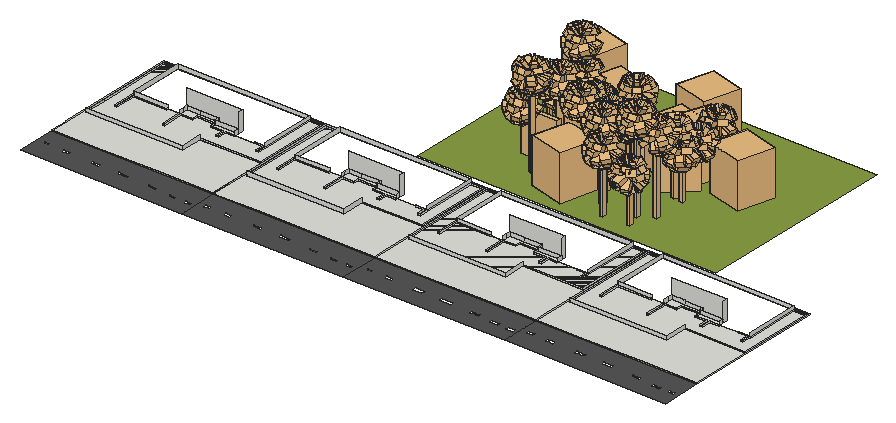
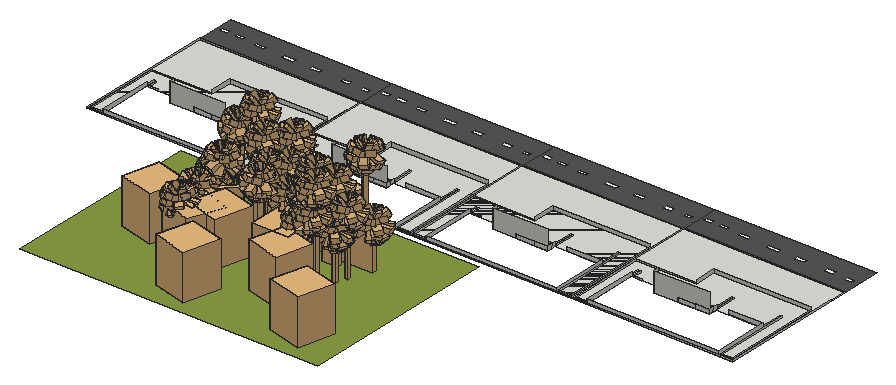
# SketchUp Ruby script. Lengths in inches.
U = 1.inch
M = Sketchup.active_model
def pt(a) = Geom::Point3d.new(a.map { |v| v * U })
def face(e, loops, mat)
  f = e.add_face(loops[0].map { |a| pt(a) })
  loops[1..].each { |l| e.add_face(l.map { |a| pt(a) }).erase! }
  f.material = f.back_material = mat if mat
  f
end
# faces: each face lists its corners as indices into pts; further lists are holes
def faces(e, pts, list, mat = nil) = list.each { |f| face(e, (f[0].is_a?(Array) ? f : [f]).map { |l| l.map { |i| pts[i] } }, mat) }
# xy, xz, yz: faces in a plane at the given z, y or x. An outline is a flat list of corners, or four numbers for a rectangle; further outlines are holes
def ring(l) = l.size == 4 ? [[l[0], l[1]], [l[2], l[1]], [l[2], l[3]], [l[0], l[3]]] : l.each_slice(2).to_a
def flat(e, list, mat, &to3) = list.each { |f| face(e, (f[0].is_a?(Array) ? f : [f]).map { |l| ring(l).map { |u, v| to3.(u, v) } }, mat) }
def xy(e, z, list, mat = nil) = flat(e, list, mat) { |x, y| [x, y, z] }
def xz(e, y, list, mat = nil) = flat(e, list, mat) { |x, z| [x, y, z] }
def yz(e, x, list, mat = nil) = flat(e, list, mat) { |y, z| [x, y, z] }
def lines(e, pts, list) = list.each { |a, b| e.add_line(pt(pts[a]), pt(pts[b])) }
# prism: a flat outline (further loops are holes) pulled along v
def prism(e, loops, v, mat = nil)
  f = face(e, loops, mat); d = Geom::Vector3d.new(v.map { |x| x * U })
  f.pushpull(f.normal.samedirection?(d) ? d.length : -d.length)
end
def box(e, o, s, mat = nil) = prism(e, [[o, [o[0] + s[0], o[1], o[2]], [o[0] + s[0], o[1] + s[1], o[2]], [o[0], o[1] + s[1], o[2]]]], [0, 0, s[2]], mat)
def at(x, y, z, deg = 0) = Geom::Transformation.translation(pt([x, y, z])) * Geom::Transformation.rotation(ORIGIN, Z_AXIS, deg.degrees)
def axes(o, x, y, z) = Geom::Transformation.new([*x, 0, *y, 0, *z, 0, *pt(o).to_a, 1])
def part(name) = M.definitions.add(name)
# library, detail: a bought-in or finely detailed component or shape, given as its bounding box
def library(name, o, s) = part(name).tap { |d| box(d.entities, o, s) }
def detail(e, o, s) = box(e.add_group.entities, o, s)
def put(e, d, t, mat = nil) = e.add_instance(d, t).tap { |i| i.material = mat if mat }
def group(e, t, mat = nil) = e.add_group.tap { |g| g.transformation = t; g.material = mat if mat }.entities
root = M.entities
M.materials.add("COCOLUMBER1").color = [119, 109, 95]
M.materials.add("Color_000").color = [255, 255, 255]
M.materials.add("[0133_Gray]").color = [86, 86, 86]
M.materials.add("[Grass Light Green]").color = [138, 158, 69]
M.materials.add("[Stone_Flagstone_Ashlar]").color = [175, 116, 102]
M.materials.add("[Tile Grey]").color = [168, 168, 168]
c1 = part("Untitled (5)")
xy(c1.entities,0,[[222.04,66.5,231.29,100.5],[222.61,182.28,236.36,226.53],[225.28,357.51,237.28,411.51],[226.57,518.17,239.57,583.92],[233.64,703.93,242.14,755.18],
  [240.05,835.03,248.8,880.53],[239.71,931.55,251.46,972.3]],"Color_000")
xy(c1.entities,0,[[[158.81,26.5625,306.06,993.3125],[226.57,518.17,239.57,583.92],[225.28,357.51,237.28,411.51],[222.61,182.28,236.36,226.53],[239.71,931.55,251.46,972.3],[233.64,703.93,242.14,755.18],[240.05,835.03,248.8,880.53],[222.04,66.5,231.29,100.5]]],"[0133_Gray]")
c2 = library("Palm frond \#1",[-21.27,-0.38,-4.44],[74.64,151.68,26.05])
c3 = part("Palm frond cluster")
put(c3.entities,c2,axes([98.98,59.12,-6.6],[-0.57786,0.81614,0],[-0.81614,-0.57786,0],[0,0,1.8876]))
put(c3.entities,c2,axes([105.83,88.13,9.87],[-0.67944,-0.73373,0],[0.7249,-0.67126,-0.15471],[0.21427,-0.19842,1.86487]))
put(c3.entities,c2,axes([73.46,76.73,-6.83],[1,0,0],[0,0.99443,-0.10543],[0,0.19901,1.87708]))
c4 = part("Palm crown")
put(c4.entities,c2,axes([108.09,116.23,112.23],[0.60444,0.79634,0.02211],[-0.38669,0.31755,-0.86581],[-0.57427,0.42444,0.41215]))
put(c4.entities,c2,axes([136.99,132.05,110.62],[-0.9152,-0.38852,0.10706],[0.08408,-0.44389,-0.89213],[0.32496,-0.66577,0.36188]))
put(c4.entities,c2,axes([122.18,113.8,111.54],[0.08804,0.99481,0.05098],[-0.50379,0.08862,-0.85927],[-0.70852,0.0412,0.41966]))
put(c4.entities,c2,axes([127.99,125.91,114.12],[-0.30715,0.21543,0.04369],[-0.00716,-0.23041,1.0858],[0.26841,0.36655,0.07955]))
put(c4.entities,c2,axes([103.59,126.54,118.32],[0.96893,0.24682,0.01605],[-0.22321,0.84461,0.48663],[0.20112,-0.89679,1.64874]))
put(c4.entities,c2,axes([132.625,118.58,110.86],[-0.79198,0.60227,0.10017],[-0.36651,-0.33776,-0.86694],[-0.4026,-0.59638,0.40255]))
put(c4.entities,c2,axes([132.69,143.375,115.86],[-0.48474,-0.87071,0.083],[0.68927,-0.43869,-0.5766],[1.01639,-0.4196,1.53425]))
put(c4.entities,c3,axes([128.89,9.89,132.21],[0.59014,0.791,-0.16144],[-0.79634,0.60321,0.04452],[0.1326,0.10229,0.98588]))
put(c4.entities,c2,axes([110.58,141.22,117.1],[0.63855,-0.76931,0.0202],[0.63758,0.51415,-0.57371],[0.8135,0.71582,1.54559]))
put(c4.entities,c2,axes([124.78,146.64,115.88],[-0.11221,-0.99112,0.07129],[0.92652,-0.13028,-0.35296],[0.67787,0.04993,1.76097]))
put(c4.entities,c2,axes([122.51,149.42,117.04],[0.39103,-0.91975,0.03404],[0.19966,0.04866,-0.97866],[0.74078,0.32113,0.1671]))
put(c4.entities,c2,axes([109.625,140.35,117.99],[0.86054,-0.50891,0.02211],[0.4462,0.77402,0.44921],[-0.46382,-0.71105,1.68592]))
put(c4.entities,c2,axes([116.71,128.1875,118.1],[0.61604,-0.07661,0.00027],[0.03235,0.25679,-0.96593],[0.09819,0.79033,0.2134]),"COCOLUMBER1")
put(c4.entities,c2,axes([106.79,121.78,118.63],[0.90526,0.41496,-0.09122],[-0.38356,0.70587,-0.59551],[-0.34491,1.08363,1.50659]))
put(c4.entities,c2,axes([127.38,115.49,111.15],[-0.41996,0.90406,0.07938],[-0.48716,-0.15078,-0.8602],[-0.63133,-0.32974,0.41534]))
put(c4.entities,c2,axes([126.87,112.82,117.51],[-0.39428,0.9188,-0.01857],[-0.74747,-0.33238,-0.57517],[-1.00919,-0.40185,1.54373]))
put(c4.entities,c2,axes([136.51,114.68,116.54],[-0.8132,0.57038,0.11567],[-0.44883,-0.74115,0.49924],[0.69933,0.66833,1.62089]))
put(c4.entities,c2,axes([139.34,132.85,114.96],[-0.95658,-0.27018,0.10937],[0.1925,-0.86734,-0.45898],[0.41314,-0.78901,1.66428]))
put(c4.entities,c2,axes([114.58,111.42,117.76],[0.273,0.96044,0.05495],[-0.82871,0.20578,0.52048],[0.92224,-0.35418,1.60843]))
put(c4.entities,c3,axes([34.06,50.17,99.19],[1,0,0],[0,0.96593,0.25882],[0,-0.25882,0.96593]))
put(c4.entities,c2,axes([129.57,143.93,113.7],[-0.59821,-0.79634,0.08934],[0.41703,-0.40458,-0.81388],[0.56418,-0.37071,0.47337]))
put(c4.entities,c2,axes([130.72,144.4375,116.95],[-0.38164,-0.91976,0.09155],[0.8496,-0.31006,0.42666],[-0.68716,0.45418,1.6984]))
put(c4.entities,c2,axes([131.04,111.78,119.35],[-0.80044,0.5994,0.00413],[-0.42618,-0.56425,-0.7071],[-0.79563,-1.07169,1.33472]))
put(c4.entities,c2,axes([110.2,144.05,126.35],[0.60643,-0.7943,0.03632],[0.64903,0.52087,0.55448],[-0.86705,-0.59022,1.56936]))
put(c4.entities,c2,axes([142.64,131.42,116.29],[-0.95847,-0.25692,0.12379],[0.28487,-0.84195,0.45823],[-0.02548,0.8956,1.66141]))
put(c4.entities,c2,axes([119.45,118.27,117.33],[0.21648,0.59293,0.03228],[-0.46829,0.12335,0.87492],[0.90601,-0.35995,0.53567]))
put(c4.entities,c2,axes([117.27,113.7,118.04],[0.23506,0.97049,-0.05375],[-0.80388,0.16302,-0.57201],[-1.03133,0.33537,1.54496]))
put(c4.entities,c2,axes([111.15,130.86,117.79],[0.59448,-0.21434,0.01115],[0.17045,0.51639,0.83922],[-0.32671,-0.8747,0.60458]))
put(c4.entities,c2,axes([131.22,120.64,116.67],[-0.51397,0.3605,0.07311],[-0.2051,-0.46687,0.86021],[0.60585,0.75173,0.55245]))
put(c4.entities,c2,axes([124.93,138.67,117.02],[-0.21153,-0.59293,0.0562],[0.56288,-0.12335,0.81728],[-0.84066,0.35995,0.63331]))
put(c4.entities,c2,axes([125.97,109.88,116.19],[-0.24621,0.96375,0.10281],[-0.94431,-0.21463,-0.24942],[-0.41209,-0.29916,1.81761]))
put(c4.entities,c2,axes([112.49,114.18,118.67],[0.68775,0.72163,-0.07906],[-0.67912,0.60109,-0.4213],[-0.48416,0.64828,1.70539]))
c5 = part("Group\#141")
put(c5.entities,c4,axes([-0.04,31.24,176.27],[0.54092,-0.14494,0],[0.14494,0.54092,0],[0,0,0.56]),"[Stone_Flagstone_Ashlar]")
g1 = group(c5.entities,at(43.85,611.85,9.84))
detail(g1,[29.01,-534.03,-9.84],[20.18,17.89,236.22])
c6 = library("Group\#112",[280.3,-607.43,-9.84],[21.76,21.76,393.7])
c7 = part("Group\#143")
put(c7.entities,c4,axes([14.65,13.97,332.76],[0.56,0,0],[0,0.56,0],[0,0,0.56]),"[Stone_Flagstone_Ashlar]")
put(c7.entities,c6,at(-205.96,691.71,9.84))
c8 = library("Group\#131",[336.49,-607.32,-9.84],[23.63,23.62,472.44])
c9 = part("Group\#142")
put(c9.entities,c4,axes([14.65,13.97,408.41],[0.56,0,0],[0,0.56,0],[0,0,0.56]),"[Stone_Flagstone_Ashlar]")
put(c9.entities,c8,axes([-199.25,630.26,9.84],[0.8099,0,0],[0,0.92,0],[0,0,1]))
c10 = part("Group\#139")
put(c10.entities,c4,axes([14.65,13.97,257.21],[0.56,0,0],[0,0.56,0],[0,0,0.56]),"[Stone_Flagstone_Ashlar]")
g2 = group(c10.entities,at(-87.26,634.75,9.84))
detail(g2,[163.83,-557.35,-9.84],[17.02,18.12,316.37])
c11 = library("Coconut",[0,0,0],[6,6,6])
c12 = part("Group\#111")
detail(c12.entities,[126.53,-566.4375,-31.76],[21.43,21.47,314.96])
c13 = part("Group\#138")
put(c13.entities,c4,axes([14.65,13.97,253.0625],[0.56,0,0],[0,0.56,0],[0,0,0.56]),"[Stone_Flagstone_Ashlar]")
put(c13.entities,c12,at(-54.86,642.08,31.76))
c14 = library("Group\#144",[-31.7,-22.28,0],[197.44,197.48,245.38])
c15 = library("Group\#217",[-86.05,-583.93,-9.84],[105.44,25.13,372.44])
c16 = part("Group\#146")
put(c16.entities,c4,axes([14.65,13.97,296.01],[0.56,0,0],[0,0.56,0],[0,0,0.56]),"[Stone_Flagstone_Ashlar]")
put(c16.entities,c15,axes([86.81,656.51,9.45],[1,0,0],[0,1,0],[0,0,0.96]))
c17 = library("Group\#137",[-509.61,-583,-9.84],[198.33,25,224.95])
c18 = part("Group\#226")
put(c18.entities,c4,axes([14.65,13.97,164.57],[0.56,0,0],[0,0.56,0],[0,0,0.56]),"[Stone_Flagstone_Ashlar]")
put(c18.entities,c17,at(588.97,655.37,9.84))
c19 = library("Group\#218",[-201.8,-584.81,-9.84],[84.72,26.88,386.61])
c20 = library("Group\#136",[-284.02,-582.12,-9.84],[34.81,21.51,275.59])
c21 = part("LANDSCAPING+Coconut+Trees")
xy(c21.entities,0,[[-341.57,-22.89,1280.875,1071.24]],"[Grass Light Green]")
put(c21.entities,c5,at(644.25,162.65,0.08,-90))
put(c21.entities,c7,at(534.68,153.22,0.24))
put(c21.entities,c9,at(627.57,68.88,0.24))
g3 = group(c21.entities,at(441.06,62.32,0.24))
put(g3,c4,axes([14.65,13.97,334.3],[0.56,0,0],[0,0.56,0],[0,0,0.56]),"[Stone_Flagstone_Ashlar]")
g4 = group(g3,at(-161.71,683.51,9.84))
detail(g4,[235.77,-605.36,-9.84],[21.85,21.73,393.32])
put(c21.entities,c10,at(507.45,-17.04,0.04))
g5 = group(c21.entities,at(384.92,163.75,0.52))
put(g5,c4,axes([14.65,13.97,253.0625],[0.56,0,0],[0,0.56,0],[0,0,0.56]),"[Stone_Flagstone_Ashlar]")
put(g5,c11,axes([78.15,82.49,296.44],[0.8993,1.53487,-0.03138],[-1.51998,0.89531,0.23158],[0.21557,-0.09025,1.76378]))
put(g5,c11,axes([79.68,82.54,287.24],[0.80142,1.36782,-0.02796],[-1.35455,0.79787,0.20637],[0.1921,-0.08042,1.57182]))
put(g5,c11,axes([77.51,71.8,291.02],[0.8993,1.53487,-0.03138],[-1.51998,0.89531,0.23158],[0.21557,-0.09025,1.76378]))
put(g5,c11,axes([86.52,87.55,293.71],[1.04679,1.7866,-0.03652],[-1.76927,1.04215,0.26956],[0.25092,-0.10505,2.05306]))
put(g5,c11,axes([92.01,70.93,291.34],[1.26662,2.16178,-0.04419],[-2.14081,1.261,0.32616],[0.30361,-0.12711,2.4842]))
put(g5,c12,at(-54.86,642.08,31.76))
put(c21.entities,c13,at(322.43,275.42,0.52,75))
put(c21.entities,c14,at(215.66,444.05,0))
put(c21.entities,c16,at(219.87,194.55,1.28))
put(c21.entities,c18,at(-99.86,200.06,0.67))
g6 = group(c21.entities,at(71.46,249.51,0.63))
put(g6,c4,axes([14.65,13.97,325.99],[0.56,0,0],[0,0.56,0],[0,0,0.56]),"[Stone_Flagstone_Ashlar]")
put(g6,c19,at(259.05,660.06,9.84))
g7 = group(c21.entities,at(290.4,300.18,0.67))
put(g7,c4,axes([14.65,13.97,214.81],[0.56,0,0],[0,0.56,0],[0,0,0.56]),"[Stone_Flagstone_Ashlar]")
put(g7,c20,at(354.13,659.23,9.84))
put(c21.entities,c14,at(768.63,688.84,0,159))
put(c21.entities,c14,at(573.53,797.54,0,75))
put(c21.entities,c9,at(18.43,450.01,0.24))
put(c21.entities,c7,at(864.55,292.18,0.24,180))
put(c21.entities,c5,at(695.7,287.05,0.08))
put(c21.entities,c5,at(135.65,408.5625,0.08))
put(c21.entities,c18,at(771.29,622.71,0.67,-134.5))
put(c21.entities,c5,at(664.4,571.51,0.08))
put(c21.entities,c16,at(563.8125,499.28,1.28,140.1))
put(c21.entities,c10,at(450.29,232.17,0.04))
put(c21.entities,c10,at(-49.04,312.68,0.04))
put(c21.entities,c10,at(52.82,431.375,0.04))
put(c21.entities,c14,at(259.5,238.44,0,-105))
put(c21.entities,c14,at(533.19,658.43,0,-105))
put(c21.entities,c5,at(-26.35,370.51,0.08))
put(c21.entities,c14,at(-48.71,797.54,0,75))
put(c21.entities,c14,at(238.42,585.39,0,75))
put(c21.entities,c14,at(891.93,658.43,0,-105))
put(c21.entities,c9,at(220.5,234.49,0.24,165))
put(c21.entities,c13,at(795.86,275.42,0.52,75))
xy(root,-16.4375,[[[276.92,393.78,1156.17,1160.85],[357.89,851.0625,357.89,1155.13,1075.21,1155.13,1075.21,851.0625,911.51,851.0625,911.51,874.25,784.44,874.25,784.44,900.375,610.53,900.375,610.53,851.0625]],[[1156.87,393.78,2036.12,1160.85],[1237.84,851.0625,1237.84,1155.13,1955.15,1155.13,1955.15,851.0625,1791.45,851.0625,1791.45,874.25,1664.38,874.25,1664.38,900.375,1490.48,900.375,1490.48,851.0625]],[[2036.8125,393.78,2916.0625,1160.85],[2117.78,851.0625,2117.78,1155.13,2835.1,1155.13,2835.1,851.0625,2671.4,851.0625,2671.4,874.25,2544.33,874.25,2544.33,900.375,2370.42,900.375,2370.42,851.0625]],[[2916.76,393.78,3796.01,1160.85],[2997.72,851.0625,2997.72,1155.13,3715.04,1155.13,3715.04,851.0625,3551.34,851.0625,3551.34,874.25,3424.27,874.25,3424.27,900.375,3250.36,900.375,3250.36,851.0625]],[[288.55,611.53,288.55,1146.63,352.17,1146.63,352.17,732.28,363.11,732.28,363.11,845.35,545.16,845.35,545.16,851.0625,610.53,851.0625,610.53,732.28,621.47,732.28,621.47,845.35,684.16,845.35,684.16,874.25,784.44,874.25,784.44,845.35,848.72,845.35,848.72,798.41,864.05,798.41,864.05,845.35,911.51,845.35,911.51,851.0625,1080.92,851.0625,1080.92,1146.63,1144.18,1146.63,1144.18,732.28,816.46,732.28,816.46,611.53],[1065.59,801.78,1080.92,845.35]],
  [[1168.49,611.53,1168.49,1146.63,1232.12,1146.63,1232.12,732.28,1243.06,732.28,1243.06,845.35,1425.1,845.35,1425.1,851.0625,1490.48,851.0625,1490.48,732.28,1501.42,732.28,1501.42,845.35,1564.1,845.35,1564.1,874.25,1664.38,874.25,1664.38,845.35,1728.67,845.35,1728.67,798.41,1744,798.41,1744,845.35,1791.45,845.35,1791.45,851.0625,1960.87,851.0625,1960.87,1146.63,2024.12,1146.63,2024.12,732.28,1696.41,732.28,1696.41,611.53],[1945.54,801.78,1960.87,845.35]],[[2048.43,611.53,2048.43,1146.63,2112.0625,1146.63,2112.0625,732.28,2123,732.28,2123,845.35,2305.05,845.35,2305.05,851.0625,2370.42,851.0625,2370.42,732.28,2381.36,732.28,2381.36,845.35,2444.05,845.35,2444.05,874.25,2544.33,874.25,2544.33,845.35,2608.61,845.35,2608.61,798.41,2623.94,798.41,2623.94,845.35,2671.4,845.35,2671.4,851.0625,2840.8125,851.0625,2840.8125,1146.63,2904.07,1146.63,2904.07,732.28,2576.35,732.28,2576.35,611.53],[2825.48,801.78,2840.8125,845.35]],[[2928.38,611.53,2928.38,1146.63,2992.01,1146.63,2992.01,732.28,3002.95,732.28,3002.95,845.35,3184.99,845.35,3184.99,851.0625,3250.36,851.0625,3250.36,732.28,3261.3,732.28,3261.3,845.35,3323.99,845.35,3323.99,874.25,3424.27,874.25,3424.27,845.35,3488.55,845.35,3488.55,798.41,3503.88,798.41,3503.88,845.35,3551.34,845.35,3551.34,851.0625,3720.76,851.0625,3720.76,1146.63,3784.01,1146.63,3784.01,732.28,3456.29,732.28,3456.29,611.53],[3705.43,801.78,3720.76,845.35]]])
xz(root,393.78,[[276.92,-16.4375,1156.17,-16.4375,1156.17,-10.51,836.67,-10.51,551.82,-12.6875,276.92,-12.6875],[1156.87,-16.4375,2036.12,-16.4375,2036.12,-10.51,1716.62,-10.51,1431.76,-12.6875,1156.87,-12.6875],[2036.8125,-16.4375,2916.0625,-16.4375,2916.0625,-10.51,2596.56,-10.51,2311.71,-12.6875,2036.8125,-12.6875],[2916.76,-16.4375,3796.01,-16.4375,3796.01,-10.51,3476.5,-10.51,3191.65,-12.6875,2916.76,-12.6875]],"[Tile Grey]")
xz(root,611.53,[[288.55,-16.4375,816.46,5.1875],[1168.49,-16.4375,1696.41,5.1875],[2048.43,-16.4375,2576.35,5.1875],[2928.38,-16.4375,3456.29,5.1875]])
xz(root,732.28,[[352.17,-16.4375,363.11,-10.51],[610.53,-16.4375,621.47,-10.51],[816.46,-16.4375,1144.18,-10.51],[1232.12,-16.4375,1243.06,-10.51],[1490.48,-16.4375,1501.42,-10.51],
  [1696.41,-16.4375,2024.12,-10.51],[2112.0625,-16.4375,2123,-10.51],[2370.42,-16.4375,2381.36,-10.51],[2576.35,-16.4375,2904.07,-10.51],[2992.01,-16.4375,3002.95,-10.51],
  [3250.36,-16.4375,3261.3,-10.51],[3456.29,-16.4375,3784.01,-10.51]])
xz(root,798.41,[[848.72,-16.4375,864.05,-10.51],[1728.67,-16.4375,1744,-10.51],[2608.61,-16.4375,2623.94,-10.51],[3488.55,-16.4375,3503.88,-10.51]])
xz(root,801.78,[[1065.59,-16.4375,1080.92,-10.51],[1945.54,-16.4375,1960.87,-10.51],[2825.48,-16.4375,2840.8125,-10.51],[3705.43,-16.4375,3720.76,-10.51]])
xz(root,845.35,[[363.11,-16.4375,545.16,-10.51],[621.47,-16.4375,684.16,-10.51],[784.44,-16.4375,848.72,-10.51],[864.05,-16.4375,911.51,-10.51],[1065.59,-16.4375,1080.92,-10.51],
  [1243.06,-16.4375,1425.1,-10.51],[1501.42,-16.4375,1564.1,-10.51],[1664.38,-16.4375,1728.67,-10.51],[1744,-16.4375,1791.45,-10.51],[1945.54,-16.4375,1960.87,-10.51],
  [2123,-16.4375,2305.05,-10.51],[2381.36,-16.4375,2444.05,-10.51],[2544.33,-16.4375,2608.61,-10.51],[2623.94,-16.4375,2671.4,-10.51],[2825.48,-16.4375,2840.8125,-10.51],
  [3002.95,-16.4375,3184.99,-10.51],[3261.3,-16.4375,3323.99,-10.51],[3424.27,-16.4375,3488.55,-10.51],[3503.88,-16.4375,3551.34,-10.51],[3705.43,-16.4375,3720.76,-10.51]])
xz(root,851.0625,[[357.89,-16.4375,545.16,5.1875],[1016.125,-16.4375,1075.21,-10.51],[1075.21,-16.4375,1080.92,-10.51],[1237.84,-16.4375,1425.1,5.1875],[1896.07,-16.4375,1955.15,-10.51],
  [1955.15,-16.4375,1960.87,-10.51],[2117.78,-16.4375,2305.05,5.1875],[2776.01,-16.4375,2835.1,-10.51],[2835.1,-16.4375,2840.8125,-10.51],[2997.72,-16.4375,3184.99,5.1875],
  [3655.96,-16.4375,3715.04,-10.51],[3715.04,-16.4375,3720.76,-10.51]])
xz(root,874.25,[[684.16,-16.4375,784.44,-10.51],[784.44,-16.4375,911.51,5.1875],[1564.1,-16.4375,1664.38,-10.51],[1664.38,-16.4375,1791.45,5.1875],[2444.05,-16.4375,2544.33,-10.51],
  [2544.33,-16.4375,2671.4,5.1875],[3323.99,-16.4375,3424.27,-10.51],[3424.27,-16.4375,3551.34,5.1875]])
xz(root,900.375,[[610.53,-16.4375,684.16,5.1875],[784.44,-16.4375,784.44,5.1875,610.53,5.1875,610.53,89.42,911.51,89.42,911.51,-16.4375],[684.16,-16.4375,784.44,5.1875],[1490.48,-16.4375,1564.1,5.1875],[1664.38,-16.4375,1664.38,5.1875,1490.48,5.1875,1490.48,89.42,1791.45,89.42,1791.45,-16.4375],
  [1564.1,-16.4375,1664.38,5.1875],[2370.42,-16.4375,2444.05,5.1875],[2544.33,-16.4375,2544.33,5.1875,2370.42,5.1875,2370.42,89.42,2671.4,89.42,2671.4,-16.4375],[2444.05,-16.4375,2544.33,5.1875],[3250.36,-16.4375,3323.99,5.1875],
  [3424.27,-16.4375,3424.27,5.1875,3250.36,5.1875,3250.36,89.42,3551.34,89.42,3551.34,-16.4375],[3323.99,-16.4375,3424.27,5.1875]])
xz(root,1146.63,[[288.55,-16.4375,352.17,-10.51],[1080.92,-16.4375,1144.18,-10.51],[1168.49,-16.4375,1232.12,-10.51],[1960.87,-16.4375,2024.12,-10.51],[2048.43,-16.4375,2112.0625,-10.51],
  [2840.8125,-16.4375,2904.07,-10.51],[2928.38,-16.4375,2992.01,-10.51],[3720.76,-16.4375,3784.01,-10.51]])
xz(root,1155.13,[[357.89,-16.4375,1075.21,5.1875],[1237.84,-16.4375,1955.15,5.1875],[2117.78,-16.4375,2835.1,5.1875],[2997.72,-16.4375,3715.04,5.1875]])
xz(root,1160.85,[[276.92,-16.4375,1156.17,-10.51],[1156.87,-16.4375,2036.12,-10.51],[2036.8125,-16.4375,2916.0625,-10.51],[2916.76,-16.4375,3796.01,-10.51]])
yz(root,276.92,[[393.78,-16.4375,393.78,-12.6875,491.47,-12.6875,491.47,-10.51,1160.85,-10.51,1160.85,-16.4375]])
yz(root,288.55,[[611.53,-16.4375,732.28,-10.51],[732.28,-16.4375,1146.63,-10.51]])
yz(root,352.17,[[732.28,-16.4375,1146.63,-10.51]])
yz(root,357.89,[[851.0625,-16.4375,1155.13,5.1875]])
yz(root,363.11,[[732.28,-16.4375,845.35,-10.51]])
yz(root,545.16,[[845.35,-16.4375,851.0625,-10.51]])
yz(root,610.53,[[732.28,-16.4375,846.1,-10.51],[846.1,-16.4375,851.0625,-10.51],[851.0625,-16.4375,874.25,5.1875],[874.25,-16.4375,900.375,5.1875]])
yz(root,621.47,[[732.28,-16.4375,845.35,-10.51]])
yz(root,684.16,[[845.35,-16.4375,846.1,-10.51],[846.1,-16.4375,874.25,-10.51]])
yz(root,784.44,[[845.35,-16.4375,846.1,-10.51],[846.1,-16.4375,874.25,-10.51],[874.25,-16.4375,892.35,5.1875],[892.35,-16.4375,900.375,5.1875]])
yz(root,816.46,[[611.53,-16.4375,732.28,5.1875]])
yz(root,848.72,[[798.41,-16.4375,845.35,-10.51]])
yz(root,864.05,[[798.41,-16.4375,845.35,-10.51]])
yz(root,911.51,[[845.35,-16.4375,846.1,-10.51],[846.1,-16.4375,851.0625,-10.51],[851.0625,-16.4375,874.25,5.1875],[874.25,-16.4375,900.375,89.42]])
yz(root,1065.59,[[801.78,-16.4375,845.35,-10.51]])
yz(root,1075.21,[[851.0625,-16.4375,1155.13,5.1875]])
yz(root,1080.92,[[801.78,-16.4375,845.35,-10.51],[851.0625,-16.4375,1146.63,-10.51]])
yz(root,1144.18,[[732.28,-16.4375,1146.63,-10.51]])
yz(root,1156.17,[[393.78,-16.4375,1160.85,-10.51]])
yz(root,1156.87,[[393.78,-16.4375,393.78,-12.6875,491.47,-12.6875,491.47,-10.51,1160.85,-10.51,1160.85,-16.4375]])
yz(root,1168.49,[[611.53,-16.4375,732.28,-10.51],[732.28,-16.4375,1146.63,-10.51]])
yz(root,1232.12,[[732.28,-16.4375,1146.63,-10.51]])
yz(root,1237.84,[[851.0625,-16.4375,1155.13,5.1875]])
yz(root,1243.06,[[732.28,-16.4375,845.35,-10.51]])
yz(root,1425.1,[[845.35,-16.4375,851.0625,-10.51]])
yz(root,1490.48,[[732.28,-16.4375,846.1,-10.51],[846.1,-16.4375,851.0625,-10.51],[851.0625,-16.4375,874.25,5.1875],[874.25,-16.4375,900.375,5.1875]])
yz(root,1501.42,[[732.28,-16.4375,845.35,-10.51]])
yz(root,1564.1,[[845.35,-16.4375,846.1,-10.51],[846.1,-16.4375,874.25,-10.51]])
yz(root,1664.38,[[845.35,-16.4375,846.1,-10.51],[846.1,-16.4375,874.25,-10.51],[874.25,-16.4375,892.35,5.1875],[892.35,-16.4375,900.375,5.1875]])
yz(root,1696.41,[[611.53,-16.4375,732.28,5.1875]])
yz(root,1728.67,[[798.41,-16.4375,845.35,-10.51]])
yz(root,1744,[[798.41,-16.4375,845.35,-10.51]])
yz(root,1791.45,[[845.35,-16.4375,846.1,-10.51],[846.1,-16.4375,851.0625,-10.51],[851.0625,-16.4375,874.25,5.1875],[874.25,-16.4375,900.375,89.42]])
yz(root,1945.54,[[801.78,-16.4375,845.35,-10.51]])
yz(root,1955.15,[[851.0625,-16.4375,1155.13,5.1875]])
yz(root,1960.87,[[801.78,-16.4375,845.35,-10.51],[851.0625,-16.4375,1146.63,-10.51]])
yz(root,2024.12,[[732.28,-16.4375,1146.63,-10.51]])
yz(root,2036.12,[[393.78,-16.4375,1160.85,-10.51]])
yz(root,2036.8125,[[393.78,-16.4375,393.78,-12.6875,491.47,-12.6875,491.47,-10.51,1160.85,-10.51,1160.85,-16.4375]])
yz(root,2048.43,[[611.53,-16.4375,732.28,-10.51],[732.28,-16.4375,1146.63,-10.51]])
yz(root,2112.0625,[[732.28,-16.4375,1146.63,-10.51]])
yz(root,2117.78,[[851.0625,-16.4375,1155.13,5.1875]])
yz(root,2123,[[732.28,-16.4375,845.35,-10.51]])
yz(root,2305.05,[[845.35,-16.4375,851.0625,-10.51]])
yz(root,2370.42,[[732.28,-16.4375,846.1,-10.51],[846.1,-16.4375,851.0625,-10.51],[851.0625,-16.4375,874.25,5.1875],[874.25,-16.4375,900.375,5.1875]])
yz(root,2381.36,[[732.28,-16.4375,845.35,-10.51]])
yz(root,2444.05,[[845.35,-16.4375,846.1,-10.51],[846.1,-16.4375,874.25,-10.51]])
yz(root,2544.33,[[845.35,-16.4375,846.1,-10.51],[846.1,-16.4375,874.25,-10.51],[874.25,-16.4375,892.35,5.1875],[892.35,-16.4375,900.375,5.1875]])
yz(root,2576.35,[[611.53,-16.4375,732.28,5.1875]])
yz(root,2608.61,[[798.41,-16.4375,845.35,-10.51]])
yz(root,2623.94,[[798.41,-16.4375,845.35,-10.51]])
yz(root,2671.4,[[845.35,-16.4375,846.1,-10.51],[846.1,-16.4375,851.0625,-10.51],[851.0625,-16.4375,874.25,5.1875],[874.25,-16.4375,900.375,89.42]])
yz(root,2825.48,[[801.78,-16.4375,845.35,-10.51]])
yz(root,2835.1,[[851.0625,-16.4375,1155.13,5.1875]])
yz(root,2840.8125,[[801.78,-16.4375,845.35,-10.51],[851.0625,-16.4375,1146.63,-10.51]])
yz(root,2904.07,[[732.28,-16.4375,1146.63,-10.51]])
yz(root,2916.0625,[[393.78,-16.4375,1160.85,-10.51]])
yz(root,2916.76,[[393.78,-16.4375,393.78,-12.6875,491.47,-12.6875,491.47,-10.51,1160.85,-10.51,1160.85,-16.4375]])
yz(root,2928.38,[[611.53,-16.4375,732.28,-10.51],[732.28,-16.4375,1146.63,-10.51]])
yz(root,2992.01,[[732.28,-16.4375,1146.63,-10.51]])
yz(root,2997.72,[[851.0625,-16.4375,1155.13,5.1875]])
yz(root,3002.95,[[732.28,-16.4375,845.35,-10.51]])
yz(root,3184.99,[[845.35,-16.4375,851.0625,-10.51]])
yz(root,3250.36,[[732.28,-16.4375,846.1,-10.51],[846.1,-16.4375,851.0625,-10.51],[851.0625,-16.4375,874.25,5.1875],[874.25,-16.4375,900.375,5.1875]])
yz(root,3261.3,[[732.28,-16.4375,845.35,-10.51]])
yz(root,3323.99,[[845.35,-16.4375,846.1,-10.51],[846.1,-16.4375,874.25,-10.51]])
yz(root,3424.27,[[845.35,-16.4375,846.1,-10.51],[846.1,-16.4375,874.25,-10.51],[874.25,-16.4375,892.35,5.1875],[892.35,-16.4375,900.375,5.1875]])
yz(root,3456.29,[[611.53,-16.4375,732.28,5.1875]])
yz(root,3488.55,[[798.41,-16.4375,845.35,-10.51]])
yz(root,3503.88,[[798.41,-16.4375,845.35,-10.51]])
yz(root,3551.34,[[845.35,-16.4375,846.1,-10.51],[846.1,-16.4375,851.0625,-10.51],[851.0625,-16.4375,874.25,5.1875],[874.25,-16.4375,900.375,89.42]])
yz(root,3705.43,[[801.78,-16.4375,845.35,-10.51]])
yz(root,3715.04,[[851.0625,-16.4375,1155.13,5.1875]])
yz(root,3720.76,[[801.78,-16.4375,845.35,-10.51],[851.0625,-16.4375,1146.63,-10.51]])
yz(root,3784.01,[[732.28,-16.4375,1146.63,-10.51]])
yz(root,3796.01,[[393.78,-16.4375,1160.85,-10.51]])
put(root,c1,axes([2012.63,624.05,-16.4375],[0,-1.45,0],[0.91021,0,0],[0,0,1]),"[0133_Gray]")
put(root,c1,axes([2892.58,624.05,-16.4375],[0,-1.45,0],[0.91021,0,0],[0,0,1]),"[0133_Gray]")
put(root,c21,at(1973.82,1220.18,-16.4375))
put(root,c1,axes([252.75,624.05,-16.4375],[0,-1.45,0],[0.91021,0,0],[0,0,1]),"[0133_Gray]")
put(root,c1,axes([1132.69,624.05,-16.4375],[0,-1.45,0],[0.91021,0,0],[0,0,1]),"[0133_Gray]")
